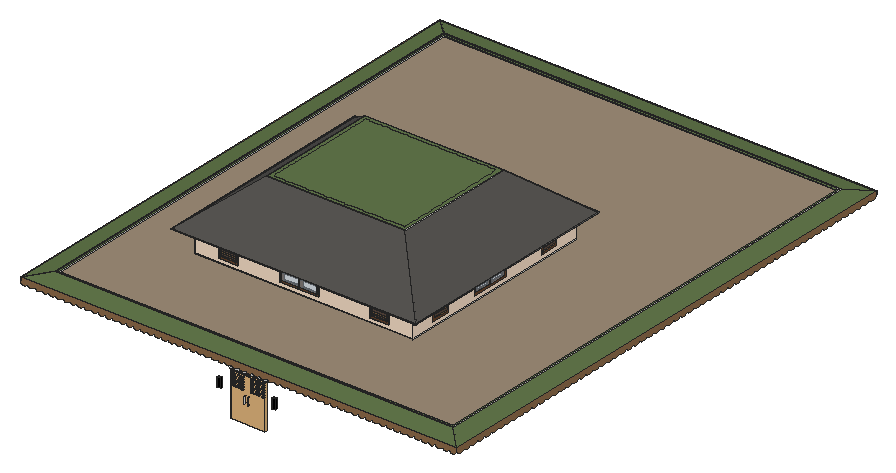
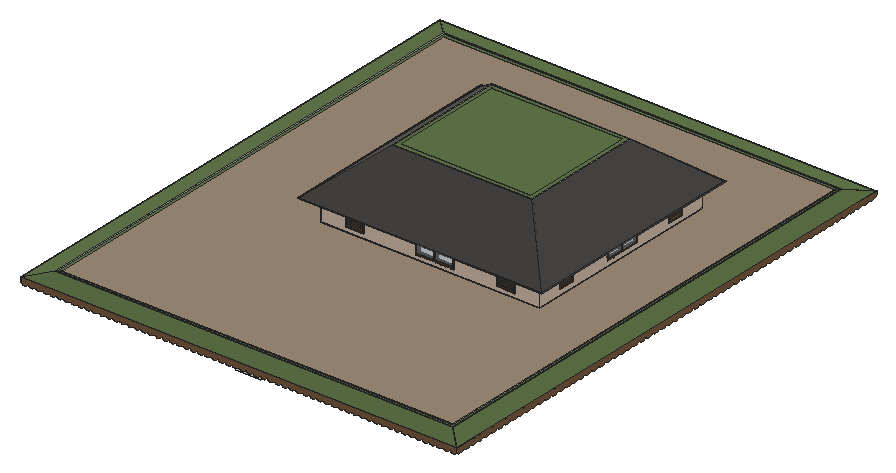
# SketchUp Ruby script. Lengths in inches.
U = 1.inch
M = Sketchup.active_model
def pt(a) = Geom::Point3d.new(a.map { |v| v * U })
def face(e, loops, mat)
  f = e.add_face(loops[0].map { |a| pt(a) })
  loops[1..].each { |l| e.add_face(l.map { |a| pt(a) }).erase! }
  f.material = f.back_material = mat if mat
  f
end
# faces: each face lists its corners as indices into pts; further lists are holes
def faces(e, pts, list, mat = nil) = list.each { |f| face(e, (f[0].is_a?(Array) ? f : [f]).map { |l| l.map { |i| pts[i] } }, mat) }
# xy, xz, yz: faces in a plane at the given z, y or x. An outline is a flat list of corners, or four numbers for a rectangle; further outlines are holes
def ring(l) = l.size == 4 ? [[l[0], l[1]], [l[2], l[1]], [l[2], l[3]], [l[0], l[3]]] : l.each_slice(2).to_a
def flat(e, list, mat, &to3) = list.each { |f| face(e, (f[0].is_a?(Array) ? f : [f]).map { |l| ring(l).map { |u, v| to3.(u, v) } }, mat) }
def xy(e, z, list, mat = nil) = flat(e, list, mat) { |x, y| [x, y, z] }
def xz(e, y, list, mat = nil) = flat(e, list, mat) { |x, z| [x, y, z] }
def yz(e, x, list, mat = nil) = flat(e, list, mat) { |y, z| [x, y, z] }
def lines(e, pts, list) = list.each { |a, b| e.add_line(pt(pts[a]), pt(pts[b])) }
# prism: a flat outline (further loops are holes) pulled along v
def prism(e, loops, v, mat = nil)
  f = face(e, loops, mat); d = Geom::Vector3d.new(v.map { |x| x * U })
  f.pushpull(f.normal.samedirection?(d) ? d.length : -d.length)
end
def box(e, o, s, mat = nil) = prism(e, [[o, [o[0] + s[0], o[1], o[2]], [o[0] + s[0], o[1] + s[1], o[2]], [o[0], o[1] + s[1], o[2]]]], [0, 0, s[2]], mat)
def at(x, y, z, deg = 0) = Geom::Transformation.translation(pt([x, y, z])) * Geom::Transformation.rotation(ORIGIN, Z_AXIS, deg.degrees)
def axes(o, x, y, z) = Geom::Transformation.new([*x, 0, *y, 0, *z, 0, *pt(o).to_a, 1])
def part(name) = M.definitions.add(name)
# library, detail: a bought-in or finely detailed component or shape, given as its bounding box
def library(name, o, s) = part(name).tap { |d| box(d.entities, o, s) }
def detail(e, o, s) = box(e.add_group.entities, o, s)
def put(e, d, t, mat = nil) = e.add_instance(d, t).tap { |i| i.material = mat if mat }
def group(e, t, mat = nil) = e.add_group.tap { |g| g.transformation = t; g.material = mat if mat }.entities
root = M.entities
M.materials.add("Brick_20_1K").color = [126, 109, 93]
M.materials.add("C01_Vanilla_Cream").color = [255, 230, 206]
M.materials.add("Glass_Basic_01").color = [161, 173, 186]
M.materials["Glass_Basic_01"].alpha = 0.57
M.materials.add("M02_Ash_Whisper").color = [196, 196, 196]
M.materials.add("M05_Graphite_Haze").color = [114, 114, 114]
M.materials.add("M07_Charcoal_Gleam").color = [58, 58, 58]
M.materials.add("M09_Shadow_Night").color = [0, 0, 0]
M.materials.add("Metal_06_1K").color = [238, 236, 231]
M.materials.add("Plaster_02_1K").color = [157, 140, 119]
M.materials.add("Plywood_01_1K").color = [125, 96, 64]
M.materials.add("Roofing_02_1K").color = [97, 118, 74]
M.materials.add("Roofing_07_1K").color = [87, 85, 82]
M.materials.add("Wood_Floor_01_1K").color = [146, 111, 76]
M.materials.add("Wood_Floor_12_1K").color = [92, 75, 65]
M.materials.add("Wood_Veneer_15_1K").color = [103, 69, 45]
c1 = part("Group\#22")
prism(c1.entities,[[[0,-12.5625,7.3125],[0,0.9375,7.3125],[0,0.9375,0],[0,0,0],[0,0,6.25],[0,-11.9375,6.25],[0,-11.9375,0],[0,-12.5625,0]]],[0.8125,0,0],"Metal_06_1K")
c2 = part("Group\#3")
box(c2.entities,[0,-3.4375,0],[6.5,3.4375,18.625],"M09_Shadow_Night")
c3 = part("Group\#26")
box(c3.entities,[0,0,0],[26,1.125,0.9375],"Wood_Floor_12_1K")
c4 = part("Group\#25")
box(c4.entities,[0,0,0],[26,1.125,0.9375],"Wood_Floor_12_1K")
c5 = part("Group\#16")
xz(c5.entities,0,[[6.84,0,8.36,0.16,9.81,0.65,11.12,1.43,12.24,2.47,13.11,3.72,13.6875,5.14,14.27,3.72,15.14,2.47,16.25,1.43,17.57,0.65,19.01,0.16,20.53,0,22.05,0.16,23.5,0.65,24.81,1.43,25.93,2.47,26.79,3.72,27.375,5.14,27.96,3.72,28.82,2.47,29.94,1.43,31.25,0.65,32.7,0.16,34.22,0,35.74,0.16,37.18,0.65,38.5,1.43,39.61,2.47,40.48,3.72,41.0625,5.14,41.64,3.72,42.51,2.47,43.63,1.43,44.94,0.65,46.39,0.16,47.91,0,49.42,0.16,50.87,0.65,52.18,1.43,53.3,2.47,54.17,3.72,54.75,5.14,55.33,3.72,56.2,2.47,57.32,1.43,58.63,0.65,60.08,0.16,61.59,0,63.11,0.16,64.56,0.65,65.87,1.43,66.99,2.47,67.86,3.72,68.4375,5.14,69.02,3.72,69.89,2.47,71,1.43,72.32,0.65,73.76,0.16,75.28,0,76.8,0.16,78.25,0.65,79.56,1.43,80.68,2.47,81.54,3.72,82.125,5.14,82.71,3.72,83.57,2.47,84.69,1.43,86,0.65,87.45,0.16,88.97,0,90.49,0.16,91.93,0.65,93.25,1.43,94.36,2.47,95.23,3.72,95.8125,5.14,96.39,3.72,97.26,2.47,98.38,1.43,99.69,0.65,101.14,0.16,102.66,0,104.17,0.16,105.62,0.65,106.93,1.43,108.05,2.47,108.92,3.72,109.5,5.14,110.08,3.72,110.95,2.47,112.07,1.43,113.38,0.65,114.83,0.16,116.34,0,117.86,0.16,119.31,0.65,120.62,1.43,121.74,2.47,122.61,3.72,123.1875,5.14,123.77,3.72,124.64,2.47,125.75,1.43,127.07,0.65,128.51,0.16,130.03,0,131.55,0.16,133,0.65,134.31,1.43,135.43,2.47,136.29,3.72,136.875,5.14,137.46,3.72,138.32,2.47,139.44,1.43,140.75,0.65,142.2,0.16,143.72,0,145.24,0.16,146.68,0.65,148,1.43,149.11,2.47,149.98,3.72,150.5625,5.14,151.14,3.72,152.01,2.47,153.13,1.43,154.44,0.65,155.89,0.16,157.41,0,158.92,0.16,160.37,0.65,161.68,1.43,162.8,2.47,163.67,3.72,164.25,5.14,164.83,3.72,165.7,2.47,166.82,1.43,168.13,0.65,169.58,0.16,171.09,0,172.61,0.16,174.06,0.65,175.37,1.43,176.49,2.47,177.36,3.72,177.9375,5.14,178.52,3.72,179.39,2.47,180.5,1.43,181.82,0.65,183.26,0.16,184.78,0,186.3,0.16,187.75,0.65,189.06,1.43,190.18,2.47,191.04,3.72,191.625,5.14,192.21,3.72,193.07,2.47,194.19,1.43,195.5,0.65,196.95,0.16,198.47,0,199.99,0.16,201.43,0.65,202.75,1.43,203.86,2.47,204.73,3.72,205.3125,5.14,205.89,3.72,206.76,2.47,207.88,1.43,209.19,0.65,210.64,0.16,212.16,0,213.67,0.16,215.12,0.65,216.43,1.43,217.55,2.47,218.42,3.72,219,5.14,219.58,3.72,220.45,2.47,221.57,1.43,222.88,0.65,224.33,0.16,225.84,0,227.36,0.16,228.81,0.65,230.12,1.43,231.24,2.47,232.11,3.72,232.6875,5.14,233.27,3.72,234.14,2.47,235.25,1.43,236.57,0.65,238.01,0.16,239.53,0,241.05,0.16,242.5,0.65,243.81,1.43,244.93,2.47,245.79,3.72,246.375,5.14,246.96,3.72,247.82,2.47,248.94,1.43,250.25,0.65,251.7,0.16,253.22,0,254.74,0.16,256.18,0.65,257.5,1.43,258.61,2.47,259.48,3.72,260.0625,5.14,260.64,3.72,261.51,2.47,262.63,1.43,263.94,0.65,265.39,0.16,266.91,0,268.42,0.16,269.87,0.65,271.18,1.43,272.3,2.47,273.17,3.72,273.75,5.14,274.33,3.72,275.2,2.47,276.32,1.43,277.63,0.65,279.08,0.16,280.59,0,282.11,0.16,283.56,0.65,284.87,1.43,285.99,2.47,286.86,3.72,287.4375,5.14,288.02,3.72,288.89,2.47,290,1.43,291.32,0.65,292.76,0.16,294.28,0,295.8,0.16,297.25,0.65,298.56,1.43,299.68,2.47,300.54,3.72,301.125,5.14,301.71,3.72,302.57,2.47,303.69,1.43,305,0.65,306.45,0.16,307.97,0,309.49,0.16,310.93,0.65,312.25,1.43,313.36,2.47,314.23,3.72,314.8125,5.14,315.39,3.72,316.26,2.47,317.38,1.43,318.69,0.65,320.14,0.16,321.66,0,323.17,0.16,324.62,0.65,325.93,1.43,327.05,2.47,327.92,3.72,328.5,5.14,329.08,3.72,329.95,2.47,331.07,1.43,332.38,0.65,333.83,0.16,335.34,0,336.86,0.16,338.31,0.65,339.62,1.43,340.74,2.47,341.61,3.72,342.1875,5.14,342.77,3.72,343.64,2.47,344.75,1.43,346.07,0.65,347.51,0.16,349.03,0,350.55,0.16,352,0.65,353.31,1.43,354.43,2.47,355.29,3.72,355.875,5.14,356.46,3.72,357.32,2.47,358.44,1.43,359.75,0.65,361.2,0.16,362.72,0,364.24,0.16,365.68,0.65,367,1.43,368.11,2.47,368.98,3.72,369.5625,5.14,370.14,3.72,371.01,2.47,372.13,1.43,373.44,0.65,374.89,0.16,376.41,0,377.92,0.16,379.37,0.65,380.68,1.43,381.8,2.47,382.67,3.72,383.25,5.14,383.83,3.72,384.7,2.47,385.82,1.43,387.13,0.65,388.58,0.16,390.09,0,391.61,0.16,393.06,0.65,394.37,1.43,395.49,2.47,396.36,3.72,396.9375,5.14,397.52,3.72,398.39,2.47,399.5,1.43,400.82,0.65,402.26,0.16,403.78,0,405.3,0.16,406.75,0.65,408.06,1.43,409.18,2.47,410.04,3.72,410.625,5.14,411.21,3.72,412.07,2.47,413.19,1.43,414.5,0.65,415.95,0.16,417.47,0,418.99,0.16,420.43,0.65,421.75,1.43,422.86,2.47,423.73,3.72,424.3125,5.14,424.89,3.72,425.76,2.47,426.88,1.43,428.19,0.65,429.64,0.16,431.16,0,432.67,0.16,434.12,0.65,435.43,1.43,436.55,2.47,437.42,3.72,438,5.14,438.58,3.72,439.45,2.47,440.57,1.43,441.88,0.65,443.33,0.16,444.84,0,446.36,0.16,447.81,0.65,449.12,1.43,450.24,2.47,451.11,3.72,451.6875,5.14,452.27,3.72,453.14,2.47,454.25,1.43,455.57,0.65,457.01,0.16,458.53,0,460.05,0.16,461.5,0.65,462.81,1.43,463.93,2.47,464.79,3.72,465.375,5.14,465.96,3.72,466.82,2.47,467.94,1.43,469.25,0.65,470.7,0.16,472.22,0,473.74,0.16,475.18,0.65,476.5,1.43,477.61,2.47,478.48,3.72,479.0625,5.14,479.64,3.72,480.51,2.47,481.63,1.43,482.94,0.65,484.39,0.16,485.91,0,487.42,0.16,488.87,0.65,490.18,1.43,491.3,2.47,492.17,3.72,492.75,5.14,493.33,3.72,494.2,2.47,495.32,1.43,496.63,0.65,498.08,0.16,499.59,0,501.11,0.16,502.56,0.65,503.87,1.43,504.99,2.47,505.86,3.72,506.4375,5.14,507.02,3.72,507.89,2.47,509,1.43,510.32,0.65,511.76,0.16,513.28,0,514.8,0.16,516.25,0.65,517.56,1.43,518.68,2.47,519.54,3.72,520.125,5.14,520.71,3.72,521.57,2.47,522.69,1.43,524,0.65,525.45,0.16,526.97,0,528.49,0.16,529.93,0.65,531.25,1.43,532.36,2.47,533.23,3.72,533.8125,5.14,534.39,3.72,535.26,2.47,536.38,1.43,537.69,0.65,539.14,0.16,540.66,0,542.17,0.16,543.62,0.65,544.93,1.43,546.05,2.47,546.92,3.72,547.5,5.14,548.08,3.72,548.95,2.47,550.07,1.43,551.38,0.65,552.83,0.16,554.34,0,555.86,0.16,557.31,0.65,558.62,1.43,559.74,2.47,560.61,3.72,561.1875,5.14,561.77,3.72,562.64,2.47,563.75,1.43,565.07,0.65,566.51,0.16,568.03,0,569.55,0.16,571,0.65,572.31,1.43,573.43,2.47,574.29,3.72,574.875,5.14,575.46,3.72,576.32,2.47,577.44,1.43,578.75,0.65,580.2,0.16,581.72,0,583.24,0.16,584.68,0.65,586,1.43,587.11,2.47,587.98,3.72,588.5625,5.14,589.14,3.72,590.01,2.47,591.13,1.43,592.44,0.65,593.89,0.16,595.41,0,596.92,0.16,598.37,0.65,599.68,1.43,600.8,2.47,601.67,3.72,602.25,5.14,602.83,3.72,603.7,2.47,604.82,1.43,606.13,0.65,607.58,0.16,609.09,0,610.61,0.16,612.06,0.65,613.37,1.43,614.49,2.47,615.36,3.72,615.9375,5.14,616.52,3.72,617.39,2.47,618.5,1.43,619.82,0.65,621.26,0.16,622.78,0,624.3,0.16,625.75,0.65,627.06,1.43,628.18,2.47,629.04,3.72,629.625,5.14,630.21,3.72,631.07,2.47,632.19,1.43,633.5,0.65,634.95,0.16,636.47,0,637.99,0.16,639.43,0.65,640.75,1.43,641.86,2.47,642.73,3.72,643.3125,5.14,643.89,3.72,644.76,2.47,645.88,1.43,647.19,0.65,648.64,0.16,650.16,0,651.67,0.16,653.12,0.65,654.43,1.43,655.55,2.47,656.42,3.72,657,5.14,657.58,3.72,658.45,2.47,659.57,1.43,660.88,0.65,662.33,0.16,663.84,0,665.36,0.16,666.81,0.65,668.12,1.43,669.24,2.47,670.11,3.72,670.6875,5.14,671.27,3.72,672.14,2.47,673.25,1.43,674.57,0.65,676.01,0.16,677.53,0,679.05,0.16,680.5,0.65,681.81,1.43,682.93,2.47,683.79,3.72,684.375,5.14,684.96,3.72,685.82,2.47,686.94,1.43,688.25,0.65,689.7,0.16,691.22,0,692.74,0.16,694.18,0.65,695.5,1.43,696.61,2.47,697.48,3.72,698.0625,5.14,698.64,3.72,699.51,2.47,700.63,1.43,701.94,0.65,703.39,0.16,704.91,0,706.42,0.16,707.87,0.65,709.18,1.43,710.3,2.47,711.17,3.72,711.75,5.14,712.33,3.72,713.2,2.47,714.32,1.43,715.63,0.65,717.08,0.16,718.59,0,720.11,0.16,721.56,0.65,722.87,1.43,723.99,2.47,724.86,3.72,725.4375,5.14,726.02,3.72,726.89,2.47,728,1.43,729.32,0.65,730.76,0.16,732.28,0,733.8,0.16,735.25,0.65,736.56,1.43,737.68,2.47,738.54,3.72,739.125,5.14,739.71,3.72,740.57,2.47,741.69,1.43,743,0.65,744.45,0.16,745.97,0,747.49,0.16,748.93,0.65,750.25,1.43,751.36,2.47,752.23,3.72,752.8125,5.14,753.39,3.72,754.26,2.47,755.38,1.43,756.69,0.65,758.14,0.16,759.66,0,761.17,0.16,762.62,0.65,763.93,1.43,765.05,2.47,765.92,3.72,766.5,5.14,767.08,3.72,767.95,2.47,769.07,1.43,770.38,0.65,771.83,0.16,773.34,0,774.86,0.16,776.31,0.65,777.62,1.43,778.74,2.47,779.61,3.72,780.1875,5.14,780.77,3.72,781.64,2.47,782.75,1.43,784.07,0.65,785.51,0.16,787.03,0,788.55,0.16,790,0.65,791.31,1.43,792.43,2.47,793.29,3.72,793.875,5.14,794.46,3.72,795.32,2.47,796.44,1.43,797.75,0.65,799.2,0.16,800.72,0,802.24,0.16,803.68,0.65,805,1.43,806.11,2.47,806.98,3.72,807.5625,5.14,808.14,3.72,809.01,2.47,810.13,1.43,811.44,0.65,812.89,0.16,814.41,0,815.92,0.16,817.37,0.65,818.68,1.43,819.8,2.47,820.67,3.72,821.25,5.14,821.83,3.72,822.7,2.47,823.82,1.43,825.13,0.65,826.58,0.16,828.09,0,829.61,0.16,831.06,0.65,832.37,1.43,833.49,2.47,834.36,3.72,834.9375,5.14,835.52,3.72,836.39,2.47,837.5,1.43,838.82,0.65,840.26,0.16,841.78,0,843.3,0.16,844.75,0.65,846.06,1.43,847.18,2.47,848.04,3.72,848.625,5.14,850,5.14,850,12,0,12,0,5.14,0.58,3.72,1.45,2.47,2.57,1.43,3.88,0.65,5.33,0.16]],"Wood_Floor_01_1K")
c6 = part("Group\#15")
xz(c6.entities,0,[[6.84,0,8.36,0.16,9.81,0.65,11.12,1.43,12.24,2.47,13.11,3.72,13.6875,5.14,14.27,3.72,15.14,2.47,16.25,1.43,17.57,0.65,19.01,0.16,20.53,0,22.05,0.16,23.5,0.65,24.81,1.43,25.93,2.47,26.79,3.72,27.375,5.14,27.96,3.72,28.82,2.47,29.94,1.43,31.25,0.65,32.7,0.16,34.22,0,35.74,0.16,37.18,0.65,38.5,1.43,39.61,2.47,40.48,3.72,41.0625,5.14,41.64,3.72,42.51,2.47,43.63,1.43,44.94,0.65,46.39,0.16,47.91,0,49.42,0.16,50.87,0.65,52.18,1.43,53.3,2.47,54.17,3.72,54.75,5.14,55.33,3.72,56.2,2.47,57.32,1.43,58.63,0.65,60.08,0.16,61.59,0,63.11,0.16,64.56,0.65,65.87,1.43,66.99,2.47,67.86,3.72,68.4375,5.14,69.02,3.72,69.89,2.47,71,1.43,72.32,0.65,73.76,0.16,75.28,0,76.8,0.16,78.25,0.65,79.56,1.43,80.68,2.47,81.54,3.72,82.125,5.14,82.71,3.72,83.57,2.47,84.69,1.43,86,0.65,87.45,0.16,88.97,0,90.49,0.16,91.93,0.65,93.25,1.43,94.36,2.47,95.23,3.72,95.8125,5.14,96.39,3.72,97.26,2.47,98.38,1.43,99.69,0.65,101.14,0.16,102.66,0,104.17,0.16,105.62,0.65,106.93,1.43,108.05,2.47,108.92,3.72,109.5,5.14,110.08,3.72,110.95,2.47,112.07,1.43,113.38,0.65,114.83,0.16,116.34,0,117.86,0.16,119.31,0.65,120.62,1.43,121.74,2.47,122.61,3.72,123.1875,5.14,123.77,3.72,124.64,2.47,125.75,1.43,127.07,0.65,128.51,0.16,130.03,0,131.55,0.16,133,0.65,134.31,1.43,135.43,2.47,136.29,3.72,136.875,5.14,137.46,3.72,138.32,2.47,139.44,1.43,140.75,0.65,142.2,0.16,143.72,0,145.24,0.16,146.68,0.65,148,1.43,149.11,2.47,149.98,3.72,150.5625,5.14,151.14,3.72,152.01,2.47,153.13,1.43,154.44,0.65,155.89,0.16,157.41,0,158.92,0.16,160.37,0.65,161.68,1.43,162.8,2.47,163.67,3.72,164.25,5.14,164.83,3.72,165.7,2.47,166.82,1.43,168.13,0.65,169.58,0.16,171.09,0,172.61,0.16,174.06,0.65,175.37,1.43,176.49,2.47,177.36,3.72,177.9375,5.14,178.52,3.72,179.39,2.47,180.5,1.43,181.82,0.65,183.26,0.16,184.78,0,186.3,0.16,187.75,0.65,189.06,1.43,190.18,2.47,191.04,3.72,191.625,5.14,192.21,3.72,193.07,2.47,194.19,1.43,195.5,0.65,196.95,0.16,198.47,0,199.99,0.16,201.43,0.65,202.75,1.43,203.86,2.47,204.73,3.72,205.3125,5.14,205.89,3.72,206.76,2.47,207.88,1.43,209.19,0.65,210.64,0.16,212.16,0,213.67,0.16,215.12,0.65,216.43,1.43,217.55,2.47,218.42,3.72,219,5.14,219.58,3.72,220.45,2.47,221.57,1.43,222.88,0.65,224.33,0.16,225.84,0,227.36,0.16,228.81,0.65,230.12,1.43,231.24,2.47,232.11,3.72,232.6875,5.14,233.27,3.72,234.14,2.47,235.25,1.43,236.57,0.65,238.01,0.16,239.53,0,241.05,0.16,242.5,0.65,243.81,1.43,244.93,2.47,245.79,3.72,246.375,5.14,246.96,3.72,247.82,2.47,248.94,1.43,250.25,0.65,251.7,0.16,253.22,0,254.74,0.16,256.18,0.65,257.5,1.43,258.61,2.47,259.48,3.72,260.0625,5.14,260.64,3.72,261.51,2.47,262.63,1.43,263.94,0.65,265.39,0.16,266.91,0,268.42,0.16,269.87,0.65,271.18,1.43,272.3,2.47,273.17,3.72,273.75,5.14,274.33,3.72,275.2,2.47,276.32,1.43,277.63,0.65,279.08,0.16,280.59,0,282.11,0.16,283.56,0.65,284.87,1.43,285.99,2.47,286.86,3.72,287.4375,5.14,288.02,3.72,288.89,2.47,290,1.43,291.32,0.65,292.76,0.16,294.28,0,295.8,0.16,297.25,0.65,298.56,1.43,299.68,2.47,300.54,3.72,301.125,5.14,301.71,3.72,302.57,2.47,303.69,1.43,305,0.65,306.45,0.16,307.97,0,309.49,0.16,310.93,0.65,312.25,1.43,313.36,2.47,314.23,3.72,314.8125,5.14,315.39,3.72,316.26,2.47,317.38,1.43,318.69,0.65,320.14,0.16,321.66,0,323.17,0.16,324.62,0.65,325.93,1.43,327.05,2.47,327.92,3.72,328.5,5.14,329.08,3.72,329.95,2.47,331.07,1.43,332.38,0.65,333.83,0.16,335.34,0,336.86,0.16,338.31,0.65,339.62,1.43,340.74,2.47,341.61,3.72,342.1875,5.14,342.77,3.72,343.64,2.47,344.75,1.43,346.07,0.65,347.51,0.16,349.03,0,350.55,0.16,352,0.65,353.31,1.43,354.43,2.47,355.29,3.72,355.875,5.14,356.46,3.72,357.32,2.47,358.44,1.43,359.75,0.65,361.2,0.16,362.72,0,364.24,0.16,365.68,0.65,367,1.43,368.11,2.47,368.98,3.72,369.5625,5.14,370.14,3.72,371.01,2.47,372.13,1.43,373.44,0.65,374.89,0.16,376.41,0,377.92,0.16,379.37,0.65,380.68,1.43,381.8,2.47,382.67,3.72,383.25,5.14,383.83,3.72,384.7,2.47,385.82,1.43,387.13,0.65,388.58,0.16,390.09,0,391.61,0.16,393.06,0.65,394.37,1.43,395.49,2.47,396.36,3.72,396.9375,5.14,397.52,3.72,398.39,2.47,399.5,1.43,400.82,0.65,402.26,0.16,403.78,0,405.3,0.16,406.75,0.65,408.06,1.43,409.18,2.47,410.04,3.72,410.625,5.14,411.21,3.72,412.07,2.47,413.19,1.43,414.5,0.65,415.95,0.16,417.47,0,418.99,0.16,420.43,0.65,421.75,1.43,422.86,2.47,423.73,3.72,424.3125,5.14,424.89,3.72,425.76,2.47,426.88,1.43,428.19,0.65,429.64,0.16,431.16,0,432.67,0.16,434.12,0.65,435.43,1.43,436.55,2.47,437.42,3.72,438,5.14,438.58,3.72,439.45,2.47,440.57,1.43,441.88,0.65,443.33,0.16,444.84,0,446.36,0.16,447.81,0.65,449.12,1.43,450.24,2.47,451.11,3.72,451.6875,5.14,452.27,3.72,453.14,2.47,454.25,1.43,455.57,0.65,457.01,0.16,458.53,0,460.05,0.16,461.5,0.65,462.81,1.43,463.93,2.47,464.79,3.72,465.375,5.14,465.96,3.72,466.82,2.47,467.94,1.43,469.25,0.65,470.7,0.16,472.22,0,473.74,0.16,475.18,0.65,476.5,1.43,477.61,2.47,478.48,3.72,479.0625,5.14,479.64,3.72,480.51,2.47,481.63,1.43,482.94,0.65,484.39,0.16,485.91,0,487.42,0.16,488.87,0.65,490.18,1.43,491.3,2.47,492.17,3.72,492.75,5.14,493.33,3.72,494.2,2.47,495.32,1.43,496.63,0.65,498.08,0.16,499.59,0,501.11,0.16,502.56,0.65,503.87,1.43,504.99,2.47,505.86,3.72,506.4375,5.14,507.02,3.72,507.89,2.47,509,1.43,510.32,0.65,511.76,0.16,513.28,0,514.8,0.16,516.25,0.65,517.56,1.43,518.68,2.47,519.54,3.72,520.125,5.14,520.71,3.72,521.57,2.47,522.69,1.43,524,0.65,525.45,0.16,526.97,0,528.49,0.16,529.93,0.65,531.25,1.43,532.36,2.47,533.23,3.72,533.8125,5.14,534.39,3.72,535.26,2.47,536.38,1.43,537.69,0.65,539.14,0.16,540.66,0,542.17,0.16,543.62,0.65,544.93,1.43,546.05,2.47,546.92,3.72,547.5,5.14,548.08,3.72,548.95,2.47,550.07,1.43,551.38,0.65,552.83,0.16,554.34,0,555.86,0.16,557.31,0.65,558.62,1.43,559.74,2.47,560.61,3.72,561.1875,5.14,561.77,3.72,562.64,2.47,563.75,1.43,565.07,0.65,566.51,0.16,568.03,0,569.55,0.16,571,0.65,572.31,1.43,573.43,2.47,574.29,3.72,574.875,5.14,575.46,3.72,576.32,2.47,577.44,1.43,578.75,0.65,580.2,0.16,581.72,0,583.24,0.16,584.68,0.65,586,1.43,587.11,2.47,587.98,3.72,588.5625,5.14,589.14,3.72,590.01,2.47,591.13,1.43,592.44,0.65,593.89,0.16,595.41,0,596.92,0.16,598.37,0.65,599.68,1.43,600.8,2.47,601.67,3.72,602.25,5.14,602.83,3.72,603.7,2.47,604.82,1.43,606.13,0.65,607.58,0.16,609.09,0,610.61,0.16,612.06,0.65,613.37,1.43,614.49,2.47,615.36,3.72,615.9375,5.14,616.52,3.72,617.39,2.47,618.5,1.43,619.82,0.65,621.26,0.16,622.78,0,624.3,0.16,625.75,0.65,627.06,1.43,628.18,2.47,629.04,3.72,629.625,5.14,630.21,3.72,631.07,2.47,632.19,1.43,633.5,0.65,634.95,0.16,636.47,0,637.99,0.16,639.43,0.65,640.75,1.43,641.86,2.47,642.73,3.72,643.3125,5.14,643.89,3.72,644.76,2.47,645.88,1.43,647.19,0.65,648.64,0.16,650.16,0,651.67,0.16,653.12,0.65,654.43,1.43,655.55,2.47,656.42,3.72,657,5.14,657.58,3.72,658.45,2.47,659.57,1.43,660.88,0.65,662.33,0.16,663.84,0,665.36,0.16,666.81,0.65,668.12,1.43,669.24,2.47,670.11,3.72,670.6875,5.14,671.27,3.72,672.14,2.47,673.25,1.43,674.57,0.65,676.01,0.16,677.53,0,679.05,0.16,680.5,0.65,681.81,1.43,682.93,2.47,683.79,3.72,684.375,5.14,684.96,3.72,685.82,2.47,686.94,1.43,688.25,0.65,689.7,0.16,691.22,0,692.74,0.16,694.18,0.65,695.5,1.43,696.61,2.47,697.48,3.72,698.0625,5.14,698.64,3.72,699.51,2.47,700.63,1.43,701.94,0.65,703.39,0.16,704.91,0,706.42,0.16,707.87,0.65,709.18,1.43,710.3,2.47,711.17,3.72,711.75,5.14,712.33,3.72,713.2,2.47,714.32,1.43,715.63,0.65,717.08,0.16,718.59,0,720.11,0.16,721.56,0.65,722.87,1.43,723.99,2.47,724.86,3.72,725.4375,5.14,726.02,3.72,726.89,2.47,728,1.43,729.32,0.65,730.76,0.16,732.28,0,733.8,0.16,735.25,0.65,736.56,1.43,737.68,2.47,738.54,3.72,739.125,5.14,739.71,3.72,740.57,2.47,741.69,1.43,743,0.65,744.45,0.16,745.97,0,747.49,0.16,748.93,0.65,750.25,1.43,751.36,2.47,752.23,3.72,752.8125,5.14,753.39,3.72,754.26,2.47,755.38,1.43,756.69,0.65,758.14,0.16,759.66,0,761.17,0.16,762.62,0.65,763.93,1.43,765.05,2.47,765.92,3.72,766.5,5.14,767.08,3.72,767.95,2.47,769.07,1.43,770.38,0.65,771.83,0.16,773.34,0,774.86,0.16,776.31,0.65,777.62,1.43,778.74,2.47,779.61,3.72,780.1875,5.14,780.77,3.72,781.64,2.47,782.75,1.43,784.07,0.65,785.51,0.16,787.03,0,788.55,0.16,790,0.65,791.31,1.43,792.43,2.47,793.29,3.72,793.875,5.14,794.46,3.72,795.32,2.47,796.44,1.43,797.75,0.65,799.2,0.16,800.72,0,802.24,0.16,803.68,0.65,805,1.43,806.11,2.47,806.98,3.72,807.5625,5.14,808.14,3.72,809.01,2.47,810.13,1.43,811.44,0.65,812.89,0.16,814.41,0,815.92,0.16,817.37,0.65,818.68,1.43,819.8,2.47,820.67,3.72,821.25,5.14,821.83,3.72,822.7,2.47,823.82,1.43,825.13,0.65,826.58,0.16,828.09,0,829.61,0.16,831.06,0.65,832.37,1.43,833.49,2.47,834.36,3.72,834.9375,5.14,835.52,3.72,836.39,2.47,837.5,1.43,838.82,0.65,840.26,0.16,841.78,0,843.3,0.16,844.75,0.65,846.06,1.43,847.18,2.47,848.04,3.72,848.625,5.14,850,5.14,850,12,0,12,0,5.14,0.58,3.72,1.45,2.47,2.57,1.43,3.88,0.65,5.33,0.16]],"Wood_Floor_01_1K")
c7 = part("Group\#18")
xy(c7.entities,0,[[0,-6,74.5,0]],"Wood_Veneer_15_1K")
xy(c7.entities,3,[[3,-6,36.25,0],[38.25,-6,71.5,0]],"Wood_Veneer_15_1K")
xy(c7.entities,25.125,[[3,-6,36.25,0],[38.25,-6,71.5,0]],"Wood_Veneer_15_1K")
xy(c7.entities,28.125,[[0,-6,74.5,0]],"Wood_Veneer_15_1K")
xz(c7.entities,-6,[[3,3,36.25,25.125],[38.25,3,71.5,25.125]],"Glass_Basic_01")
xz(c7.entities,-6,[[[0,0,74.5,28.125],[38.25,3,71.5,25.125],[3,3,36.25,25.125]]],"Wood_Veneer_15_1K")
xz(c7.entities,0,[[[0,0,74.5,28.125],[3,3,36.25,25.125],[38.25,3,71.5,25.125]]],"Wood_Veneer_15_1K")
yz(c7.entities,0,[[-6,0,0,28.125]],"Wood_Veneer_15_1K")
yz(c7.entities,3,[[-6,3,0,25.125]],"Wood_Veneer_15_1K")
yz(c7.entities,36.25,[[-6,3,0,25.125]],"Wood_Veneer_15_1K")
yz(c7.entities,38.25,[[-6,3,0,25.125]],"Wood_Veneer_15_1K")
yz(c7.entities,71.5,[[-6,3,0,25.125]],"Wood_Veneer_15_1K")
yz(c7.entities,74.5,[[-6,0,0,28.125]],"Wood_Veneer_15_1K")
c8 = part("Group\#17")
xy(c8.entities,0,[[0,0,3,36]],"Wood_Veneer_15_1K")
xy(c8.entities,3,[[0,3,3,33]],"Wood_Veneer_15_1K")
xy(c8.entities,25.125,[[0,3,3,33]],"Wood_Veneer_15_1K")
xy(c8.entities,28.125,[[0,0,3,36]],"Wood_Veneer_15_1K")
xz(c8.entities,0,[[0,0,3,28.125]],"Wood_Veneer_15_1K")
xz(c8.entities,3,[[0,3,3,25.125]],"Wood_Veneer_15_1K")
xz(c8.entities,33,[[0,3,3,25.125]],"Wood_Veneer_15_1K")
xz(c8.entities,36,[[0,0,3,28.125]],"Wood_Veneer_15_1K")
yz(c8.entities,0,[[[0,0,36,28.125],[3,3,33,25.125]]],"Wood_Veneer_15_1K")
yz(c8.entities,3,[[3,3,33,6.4],[3,9.79,33,13.24],[3,17.2,33,21.38]],"Plywood_01_1K")
yz(c8.entities,3,[[3,6.4,33,9.79],[3,13.24,33,17.2],[3,21.38,33,25.125]],"Wood_Floor_12_1K")
yz(c8.entities,3,[[[0,0,36,28.125],[3,3,33,25.125]]],"Wood_Veneer_15_1K")
xy(root,126,[[2773.48,806.69,2845.48,815.69],[2635.48,935.69,2641.48,983.69],[2977.48,935.69,2983.48,983.69],[2773.48,983.69,2845.48,989.69],[3134.81,983.69,3170.57,989.69],
  [2515.48,989.69,2521.48,1013.69],[2532.36,1061.69,2562.36,1067.69],[2983.48,1081.39,2989.48,1129.39],[2434.48,1097.3,2443.48,1133.3],[2563.48,1169.69,2569.48,1217.69],
  [3021.96,1247.69,3069.96,1253.69],[3097.48,1256.05,3103.48,1280.05],[2785.48,1373.69,2833.48,1379.69],[2434.48,1412.46,2443.48,1460.46],[2929.48,1425.125,2935.48,1534.97],
  [2683.48,1448.15,2689.48,1496.15],[2689.48,1571.69,2731.48,1577.69],[2888.46,1571.69,2924.46,1577.69],[2937.08,1571.69,2967.08,1577.69],[2605.48,1615.16,2611.48,1641.35],
  [3001.48,1619.95,3007.48,1655.95],[2504.32,1667.69,2540.32,1673.69],[2615.5625,1667.69,2645.5625,1673.69],[2968.3,1667.69,2998.3,1673.69],[2809.48,1745.69,2857.48,1751.69]],"M02_Ash_Whisper")
xy(root,132,[[2989.48,983.69,3019.48,989.69]],"M02_Ash_Whisper")
xy(root,168,[[[2434.48,806.69,3208.48,1751.69],[2569.48,989.69,2983.48,1373.69],[2641.48,815.69,2977.48,983.69],[2935.48,1379.69,3199.48,1571.69],[2443.48,1379.69,2683.48,1571.69],[2689.48,1379.69,2929.48,1571.69],[2983.48,815.69,3199.48,983.69],[2443.48,815.69,2443.48,983.69,2521.48,983.69,2521.48,1061.69,2563.48,1061.69,2563.48,983.69,2635.48,983.69,2635.48,815.69],[2989.48,1079.69,3199.48,1247.69],[3007.48,1577.69,3199.48,1745.69],[2737.48,1577.69,2929.48,1745.69],[2443.48,1169.69,2563.48,1373.69],[2443.48,1577.69,2605.48,1667.69],[2989.48,1253.69,3097.48,1373.69],[2443.48,1673.69,2605.48,1745.69],[2443.48,1067.69,2563.48,1163.69],[3103.48,1253.69,3199.48,1373.69],[2611.48,1577.69,2731.48,1667.69],[2989.48,989.69,3097.48,1073.69],[2611.48,1673.69,2731.48,1745.69],[3103.48,989.69,3199.48,1073.69],[2935.48,1577.69,3001.48,1667.69],[2443.48,989.69,2515.48,1061.69],[2935.48,1673.69,3001.48,1745.69]]],"M02_Ash_Whisper")
xz(root,1577.69,[[2689.48,126,2731.48,168]],"M02_Ash_Whisper")
detail(root,[2776.48,805.17,39],[66,4.96,84])
put(root,c1,axes([2805.12,806.69,87.71],[1,0,0],[0,0,1],[0,-0.65,0]),"Brick_20_1K")
put(root,c1,axes([2812.31,806.69,87.71],[1,0,0],[0,0,1],[0,-0.65,0]),"Brick_20_1K")
put(root,c2,at(2752.3125,806.69,85.93))
put(root,c2,at(2858.875,806.69,85.93))
put(root,c3,at(2776.48,805.12,97.78),"Brick_20_1K")
put(root,c3,at(2816.73,805.12,97.78),"Brick_20_1K")
put(root,c3,at(2776.48,805.12,102.13),"Brick_20_1K")
put(root,c3,at(2816.73,805.12,102.13),"Brick_20_1K")
put(root,c3,at(2776.48,805.12,106.48),"Brick_20_1K")
put(root,c3,at(2816.73,805.12,106.48),"Brick_20_1K")
put(root,c3,at(2776.48,805.12,110.83),"Brick_20_1K")
put(root,c3,at(2816.73,805.12,110.83),"Brick_20_1K")
put(root,c4,at(2776.48,805.12,115.18),"Brick_20_1K")
put(root,c4,at(2816.73,805.12,115.18),"Brick_20_1K")
put(root,c3,at(2776.48,805.12,119.53),"Brick_20_1K")
put(root,c3,at(2816.73,805.12,119.53),"Brick_20_1K")
put(root,c5,at(2396.48,1789.69,156),"Wood_Floor_01_1K")
put(root,c6,axes([3246.48,1789.69,156],[0,-1.20118,0],[1,0,0],[0,0,1]),"Wood_Floor_01_1K")
put(root,c6,axes([2396.48,1789.69,156],[0,-1.20118,0],[1,0,0],[0,0,1]),"Wood_Floor_01_1K")
put(root,c5,at(2396.48,768.69,156),"Wood_Floor_01_1K")
g1 = group(root,at(2983.48,806.69,168))
xy(g1,-6,[[[-540,9,216,939],[-420,183,6,573]]])
xy(g1,0,[[-549,0,225,9],[-549,9,-540,939],[[-540,9,216,939],[-420,183,6,573]],[216,9,225,573],[-420,183,-414,567],
  [0,183,6,567],[-420,567,6,573],[216,573,225,945],[-549,939,216,945]])
xy(g1,2,[[[-543,6,219,939],[-420,177,6,573]]])
xy(g1,6,[[[-543,6,219,939],[-420,177,6,573]]],"Plaster_02_1K")
xy(g1,6,[[-543,0,-543,6,219,6,219,945,225,945,225,0]],"Roofing_02_1K")
xy(g1,6.67,[[-549,0,-549,945,219,945,219,939,-543,939,-543,0]],"Roofing_02_1K")
xz(g1,0,[[-549,0,225,2.78]])
xz(g1,0,[[-549,2.78,225,2.78,225,6,-543,6,-543,6.67,-549,6.67]],"M05_Graphite_Haze")
xz(g1,9,[[-540,-6,216,0]])
xz(g1,177,[[-420,2,0,6],[0,2,6,6]])
xz(g1,183,[[-420,-6,6,0],[-414,0,0,2]])
xz(g1,567,[[-414,0,0,2]])
xz(g1,573,[[-420,-6,6,0],[-420,2,-414,6],[-414,2,0,6],[0,2,6,6]])
xz(g1,939,[[-540,-6,216,0],[-543,6,219,6.67]])
xz(g1,945,[[-549,0,-549,6.67,219,6.67,219,6,225,6,225,0]],"M05_Graphite_Haze")
yz(g1,-549,[[0,4,945,6.67]],"M05_Graphite_Haze")
yz(g1,-543,[[0,6,6,6.67],[6,6,939,6.67]])
yz(g1,-540,[[9,-6,939,0]])
yz(g1,-420,[[183,-6,573,0],[177,2,183,6],[183,2,573,6]])
yz(g1,-414,[[183,0,567,2]])
yz(g1,0,[[183,0,567,2]])
yz(g1,6,[[183,-6,573,0],[177,2,573,6]])
yz(g1,216,[[9,-6,573,0],[573,-6,939,0]])
yz(g1,219,[[939,6,945,6.67]])
yz(g1,225,[[0,0,945,6]],"M05_Graphite_Haze")
p = [[219,939,2],[219,939,6],[-543,6,2],[-543,6,6],[-543,939,2],[-543,939,6],
  [219,6,2],[219,6,6]]
lines(g1,p,[[0,1],[2,3],[4,5],[6,7]])
g2 = group(g1,at(-549,0,0))
xy(g2,0,[[-38,-38,812,0],[774,0,774,945,-38,945,-38,983,812,983,812,0],[[-38,0,774,945],[134.07,183,549,567]]],"Wood_Floor_01_1K")
xy(g2,2.1,[[[0,0,774,945],[134.07,183,549,567]]],"Plaster_02_1K")
xz(g2,0,[[0,2.1,774,7]])
xz(g2,183,[[134.07,0,549,2.1]],"Plaster_02_1K")
xz(g2,567,[[134.07,0,549,2.1]],"Plaster_02_1K")
xz(g2,945,[[0,2.1,774,7]])
yz(g2,0,[[0,2.1,945,7]])
yz(g2,134.07,[[183,0,567,2.1]],"Plaster_02_1K")
yz(g2,549,[[183,0,567,2.1]],"Plaster_02_1K")
yz(g2,774,[[0,2.1,945,7]])
yz(g2,774,[[0,0,945,2.1]],"M07_Charcoal_Gleam")
p = [[812,-38,0],[774,0,7],[0,0,7],[-38,-38,0],[-38,0,0],[-38,-35.3125,0],
  [0,945,7],[-38,983,0],[-38,945,0],[812,983,0],[774,945,7],[812,0,0]]
faces(g2,p,[[0,1,2,3],[4,5,3,2,6,7,8],[9,10,1,0,11],[7,6,10,9]],"Roofing_02_1K")
g3 = group(g1,at(-549,0,0))
xy(g3,0,[[-38,0,0,939]],"M07_Charcoal_Gleam")
p = [[0,0,2.78],[0,0,0],[-38,983,0],[-38,939,0],[-38,-38,0],[0,0,7],
  [0,945,7],[-38,0,0]]
lines(g3,p,[[0,1],[2,3],[4,5],[5,6],[6,2],[7,4]])
g4 = group(g1,at(-420,177,2))
xy(g4,0,[[[0,0,426,396],[6,6,420,390]]])
xy(g4,12,[[167.19,0,241.69,6],[0,156.6875,6,231.1875],[166.64,390,241.14,396]])
xy(g4,12,[[48,0,84,6],[342,0,378,6],[0,48,6,84],[0,312,6,348],[48,390,84,396],
  [342,390,378,396]],"C01_Vanilla_Cream")
xy(g4,13.125,[[420,150.58,426,225.08]])
xy(g4,13.125,[[420,48,426,84],[420,312,426,348]],"C01_Vanilla_Cream")
xy(g4,40.125,[[167.19,0,241.69,6],[0,156.6875,6,231.1875],[166.64,390,241.14,396]])
xy(g4,40.125,[[48,0,84,6],[342,0,378,6],[0,48,6,84],[0,312,6,348],[48,390,84,396],
  [342,390,378,396]],"C01_Vanilla_Cream")
xy(g4,41.25,[[420,150.58,426,225.08]])
xy(g4,41.25,[[420,48,426,84],[420,312,426,348]],"C01_Vanilla_Cream")
xy(g4,48,[[[-25,-25,451,421],[0,0,426,396]]],"Wood_Floor_01_1K")
xy(g4,48.6875,[[[-24.73,-24.73,450.73,420.73],[-24.36,-24.36,450.36,420.36]]],"M05_Graphite_Haze")
xy(g4,49,[[[0,0,426,396],[6,6,420,390]]])
xy(g4,49,[[[-25,-25,451,421],[-24.73,-24.73,450.73,420.73]],[[-24.36,-24.36,450.36,420.36],[0,0,426,396]]],"M05_Graphite_Haze")
xz(g4,-25,[[-25,48,451,49]],"M05_Graphite_Haze")
xz(g4,-24.73,[[-24.73,48.6875,450.73,49]],"M05_Graphite_Haze")
xz(g4,-24.36,[[-24.36,48.6875,450.36,49]],"M05_Graphite_Haze")
xz(g4,0,[[0,48,426,49]])
xz(g4,0,[[[0,0,426,48],[167.19,12,241.69,40.125],[48,12,84,40.125],[342,12,378,40.125]]],"C01_Vanilla_Cream")
xz(g4,6,[[[6,0,420,49],[167.19,12,241.69,40.125],[48,12,84,40.125],[342,12,378,40.125]]])
xz(g4,48,[[0,12,6,40.125],[420,13.125,426,41.25]],"C01_Vanilla_Cream")
xz(g4,84,[[0,12,6,40.125],[420,13.125,426,41.25]],"C01_Vanilla_Cream")
xz(g4,150.58,[[420,13.125,426,41.25]])
xz(g4,156.6875,[[0,12,6,40.125]])
xz(g4,225.08,[[420,13.125,426,41.25]])
xz(g4,231.1875,[[0,12,6,40.125]])
xz(g4,312,[[0,12,6,40.125],[420,13.125,426,41.25]],"C01_Vanilla_Cream")
xz(g4,348,[[0,12,6,40.125],[420,13.125,426,41.25]],"C01_Vanilla_Cream")
xz(g4,390,[[[6,0,420,49],[166.64,12,241.14,40.125],[342,12,378,40.125],[48,12,84,40.125]]])
xz(g4,396,[[0,48,426,49]])
xz(g4,396,[[[0,0,426,48],[166.64,12,241.14,40.125],[342,12,378,40.125],[48,12,84,40.125]]],"C01_Vanilla_Cream")
xz(g4,420.36,[[-24.36,48.6875,450.36,49]],"M05_Graphite_Haze")
xz(g4,420.73,[[-24.73,48.6875,450.73,49]],"M05_Graphite_Haze")
xz(g4,421,[[-25,48,451,49]],"M05_Graphite_Haze")
yz(g4,-25,[[-25,48,421,49]],"M05_Graphite_Haze")
yz(g4,-24.73,[[-24.73,48.6875,420.73,49]],"M05_Graphite_Haze")
yz(g4,-24.36,[[-24.36,48.6875,420.36,49]],"M05_Graphite_Haze")
yz(g4,0,[[0,48,396,49]])
yz(g4,0,[[[0,0,396,48],[156.6875,12,231.1875,40.125],[48,12,84,40.125],[312,12,348,40.125]]],"C01_Vanilla_Cream")
yz(g4,6,[[[6,0,390,49],[156.6875,12,231.1875,40.125],[48,12,84,40.125],[312,12,348,40.125]]])
yz(g4,48,[[0,12,6,40.125],[390,12,396,40.125]],"C01_Vanilla_Cream")
yz(g4,84,[[0,12,6,40.125],[390,12,396,40.125]],"C01_Vanilla_Cream")
yz(g4,166.64,[[390,12,396,40.125]])
yz(g4,167.19,[[0,12,6,40.125]])
yz(g4,241.14,[[390,12,396,40.125]])
yz(g4,241.69,[[0,12,6,40.125]])
yz(g4,342,[[0,12,6,40.125],[390,12,396,40.125]],"C01_Vanilla_Cream")
yz(g4,378,[[0,12,6,40.125],[390,12,396,40.125]],"C01_Vanilla_Cream")
yz(g4,420,[[[6,0,390,49],[150.58,13.125,225.08,41.25],[48,13.125,84,41.25],[312,13.125,348,41.25]]])
yz(g4,426,[[0,48,396,49]])
yz(g4,426,[[[0,0,396,48],[150.58,13.125,225.08,41.25],[48,13.125,84,41.25],[312,13.125,348,41.25]]],"C01_Vanilla_Cream")
yz(g4,450.36,[[-24.36,48.6875,420.36,49]],"M05_Graphite_Haze")
yz(g4,450.73,[[-24.73,48.6875,420.73,49]],"M05_Graphite_Haze")
yz(g4,451,[[-25,48,421,49]],"M05_Graphite_Haze")
put(g4,c7,at(167.19,6,12))
put(g4,c7,at(420,150.58,13.125,90))
put(g4,c7,at(241.14,390,12,-180))
put(g4,c7,at(6,231.1875,12,-90))
g5 = group(g4,at(423,48,13.125))
xy(g5,0,[[0,0,3,36]],"Wood_Veneer_15_1K")
xy(g5,3,[[0,3,3,33]],"Wood_Veneer_15_1K")
xy(g5,25.125,[[0,3,3,33]],"Wood_Veneer_15_1K")
xy(g5,28.125,[[0,0,3,36]],"Wood_Veneer_15_1K")
xz(g5,0,[[0,0,3,28.125]],"Wood_Veneer_15_1K")
xz(g5,3,[[0,3,3,25.125]],"Wood_Veneer_15_1K")
xz(g5,33,[[0,3,3,25.125]],"Wood_Veneer_15_1K")
xz(g5,36,[[0,0,3,28.125]],"Wood_Veneer_15_1K")
yz(g5,0,[[[0,0,36,28.125],[3,3,33,25.125]]],"Wood_Veneer_15_1K")
yz(g5,3,[[3,3,33,6.4],[3,9.79,33,13.24],[3,17.2,33,21.38]],"Plywood_01_1K")
yz(g5,3,[[3,6.4,33,9.79],[3,13.24,33,17.2],[3,21.38,33,25.125]],"Wood_Floor_12_1K")
yz(g5,3,[[[0,0,36,28.125],[3,3,33,25.125]]],"Wood_Veneer_15_1K")
put(g4,c8,at(423,312,13.125))
put(g4,c8,at(378,393,12,90))
put(g4,c8,at(84,393,12,90))
put(g4,c8,at(48,3,12,-90))
put(g4,c8,at(342,3,12,-90))
put(g4,c8,at(3,348,12,-180))
put(g4,c8,at(3,84,12,-180))
g6 = group(root,at(2569.48,989.69,218))
xy(g6,1,[[-30,-30,444,414]])
xy(g6,82.1875,[[72,72,342,312]])
xy(g6,84,[[[72,72,342,312],[79.34,79.34,334.66,304.66]],[79.34,79.34,334.66,304.66]],"Roofing_02_1K")
xz(g6,72,[[72,82.1875,342,84]])
xz(g6,312,[[72,82.1875,342,84]])
yz(g6,72,[[72,82.1875,312,84]])
yz(g6,342,[[72,82.1875,312,84]])
p = [[444,-30,1],[342,72,84],[72,72,84],[-30,-30,1],[-30,414,1],[72,312,84],
  [444,414,1],[342,312,84],[0,0,0],[0,384,0],[414,0,0],[414,384,0],
  [420,-6,0],[420,390,0],[-6,390,0],[-6,-6,0]]
faces(g6,p,[[0,1,2,3],[4,3,2,5],[6,7,1,0],[4,5,7,6]],"Roofing_07_1K")
lines(g6,p,[[8,9],[10,8],[11,10],[9,11],[12,13],[13,14],[14,15],[15,12]])
